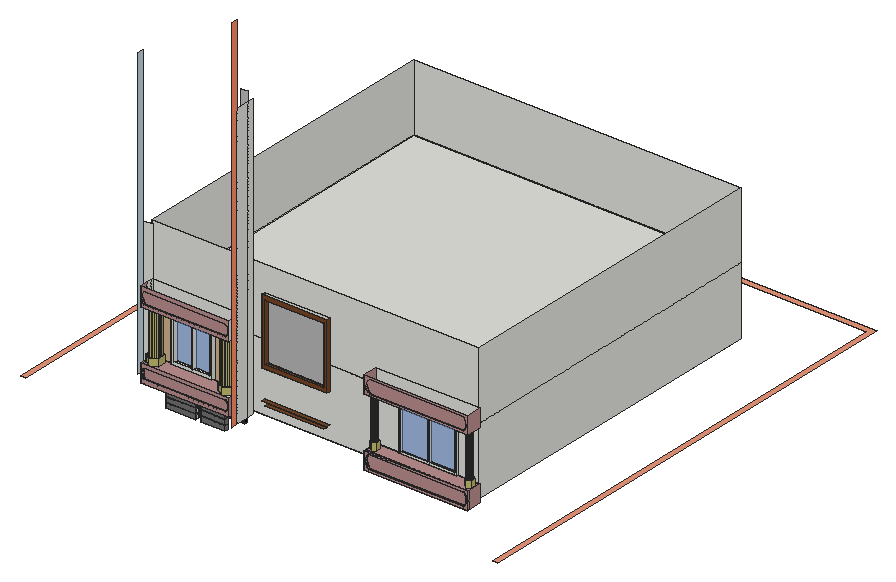
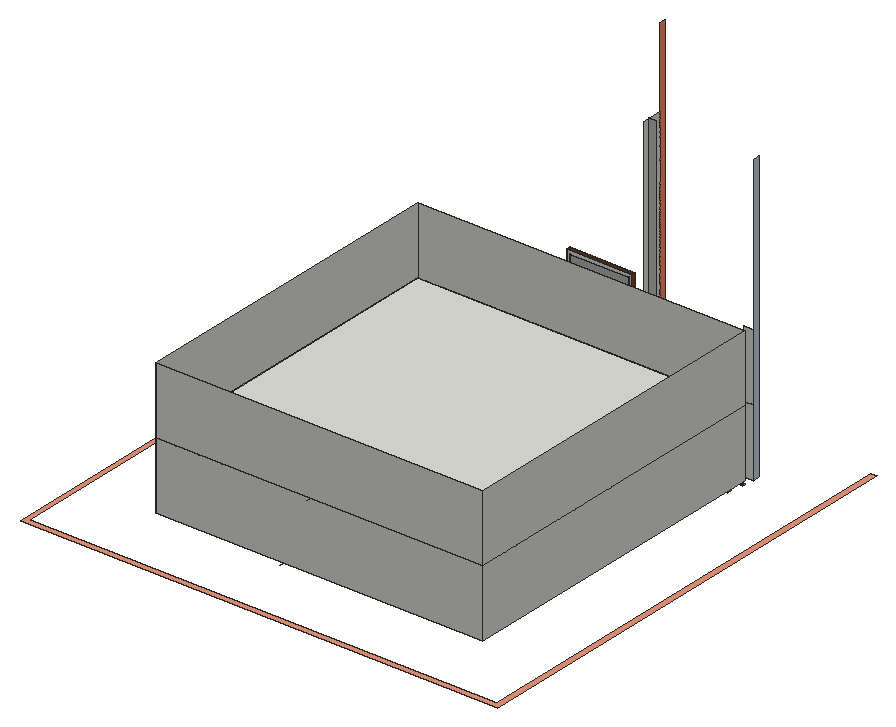
# SketchUp Ruby script. Lengths in inches.
U = 1.inch
M = Sketchup.active_model
def pt(a) = Geom::Point3d.new(a.map { |v| v * U })
def face(e, loops, mat)
  f = e.add_face(loops[0].map { |a| pt(a) })
  loops[1..].each { |l| e.add_face(l.map { |a| pt(a) }).erase! }
  f.material = f.back_material = mat if mat
  f
end
# faces: each face lists its corners as indices into pts; further lists are holes
def faces(e, pts, list, mat = nil) = list.each { |f| face(e, (f[0].is_a?(Array) ? f : [f]).map { |l| l.map { |i| pts[i] } }, mat) }
# xy, xz, yz: faces in a plane at the given z, y or x. An outline is a flat list of corners, or four numbers for a rectangle; further outlines are holes
def ring(l) = l.size == 4 ? [[l[0], l[1]], [l[2], l[1]], [l[2], l[3]], [l[0], l[3]]] : l.each_slice(2).to_a
def flat(e, list, mat, &to3) = list.each { |f| face(e, (f[0].is_a?(Array) ? f : [f]).map { |l| ring(l).map { |u, v| to3.(u, v) } }, mat) }
def xy(e, z, list, mat = nil) = flat(e, list, mat) { |x, y| [x, y, z] }
def xz(e, y, list, mat = nil) = flat(e, list, mat) { |x, z| [x, y, z] }
def yz(e, x, list, mat = nil) = flat(e, list, mat) { |y, z| [x, y, z] }
def lines(e, pts, list) = list.each { |a, b| e.add_line(pt(pts[a]), pt(pts[b])) }
# prism: a flat outline (further loops are holes) pulled along v
def prism(e, loops, v, mat = nil)
  f = face(e, loops, mat); d = Geom::Vector3d.new(v.map { |x| x * U })
  f.pushpull(f.normal.samedirection?(d) ? d.length : -d.length)
end
def box(e, o, s, mat = nil) = prism(e, [[o, [o[0] + s[0], o[1], o[2]], [o[0] + s[0], o[1] + s[1], o[2]], [o[0], o[1] + s[1], o[2]]]], [0, 0, s[2]], mat)
def at(x, y, z, deg = 0) = Geom::Transformation.translation(pt([x, y, z])) * Geom::Transformation.rotation(ORIGIN, Z_AXIS, deg.degrees)
def axes(o, x, y, z) = Geom::Transformation.new([*x, 0, *y, 0, *z, 0, *pt(o).to_a, 1])
def part(name) = M.definitions.add(name)
# library, detail: a bought-in or finely detailed component or shape, given as its bounding box
def library(name, o, s) = part(name).tap { |d| box(d.entities, o, s) }
def detail(e, o, s) = box(e.add_group.entities, o, s)
def put(e, d, t, mat = nil) = e.add_instance(d, t).tap { |i| i.material = mat if mat }
def group(e, t, mat = nil) = e.add_group.tap { |g| g.transformation = t; g.material = mat if mat }.entities
root = M.entities
M.materials.add("[0014_DarkSalmon]").color = [233, 150, 122]
M.materials.add("[0035_Tan]").color = [210, 180, 140]
M.materials.add("[0057_DarkKhaki]").color = [189, 183, 107]
M.materials.add("[0119_RosyBrown]").color = [188, 143, 143]
M.materials.add("[0131_Silver]").color = [192, 192, 192]
M.materials.add("[Color B03]").color = [255, 140, 101]
M.materials.add("[Color M05]").color = [114, 114, 114]
M.materials.add("[Color M09]").color = [0, 0, 0]
M.materials.add("[Mirror 01]").color = [185, 185, 185]
M.materials.add("[Mirror 02]").color = [229, 229, 229]
M.materials.add("[Terrazzo Light Blue]").color = [196, 214, 227]
M.materials.add("[Translucent Glass Blue]").color = [100, 149, 237]
M.materials["[Translucent Glass Blue]"].alpha = 0.5
M.materials.add("[Wood Veneer 01]").color = [120, 70, 37]
xy(root,81.75,[[173.97,107.37,183.17,113.37],[183.17,107.37,226.48,113.37]])
xy(root,81.9375,[[235.11,107.37,278.99,113.37]])
xy(root,90.5625,[[173.97,107.37,226.48,113.37]])
xy(root,90.75,[[235.11,107.37,278.99,113.37]],"[Color M05]")
xy(root,91.5625,[[173.97,107.37,183.17,113.37],[183.17,107.37,226.48,113.37]])
xy(root,91.6875,[[235.11,107.37,278.99,113.37]])
xy(root,100.375,[[173.97,107.37,226.48,113.37]])
xy(root,100.5,[[235.11,107.37,278.99,113.37]],"[Color M05]")
xy(root,101.375,[[173.97,107.37,183.17,113.37],[183.17,107.37,226.48,113.37]])
xy(root,101.4375,[[235.11,107.37,278.99,113.37]])
xy(root,101.48,[[278.99,113.37,309.83,116.37]],"[Color M09]")
xy(root,103.06,[[278.99,113.37,309.83,116.37]],"[Color M09]")
xy(root,105.17,[[143.99,113.37,173.97,116.37]],"[Color M09]")
xy(root,106.75,[[143.99,113.37,173.97,116.37]],"[Color M09]")
xy(root,110.1875,[[173.97,107.37,226.48,113.37]])
xy(root,110.25,[[235.11,107.37,278.99,113.37]])
xy(root,111.1875,[[173.97,107.37,183.17,113.37],[183.17,107.37,226.48,113.37],[235.11,107.37,278.99,113.37]])
xy(root,111.39,[[588.01,113.37,626.32,116.37],[629.68,113.37,664.64,116.37]])
xy(root,114.39,[[585.01,113.37,667.64,116.37]])
xy(root,120,[[173.97,107.37,174.52,116.37],[174.52,107.37,226.48,107.37,226.48,110.37,235.11,110.37,235.11,113.37,278.99,113.37,278.99,116.37,174.52,116.37],[235.11,107.37,278.99,113.37],[142.36,113.37,143.68,116.37],[309.83,113.37,312.71,116.37],
  [134.37,125.37,716.37,707.37]])
xy(root,120,[[0,0,9,0,9,832.73,841.73,832.73,841.73,0,850.73,0,850.73,841.73,0,841.73]],"[0014_DarkSalmon]")
xy(root,120,[[143.68,89.37,173.97,116.37],[173.97,89.37,174.52,107.37],[174.52,89.37,174.52,107.37,226.48,107.37,226.48,110.37,235.11,110.37,235.11,107.37,278.99,107.37,278.99,89.37],[278.99,89.37,299.74,116.37],[540.59,89.37,725.37,92.37],
  [540.59,92.37,725.37,116.37]],"[0119_RosyBrown]")
xy(root,123,[[548.74,89.37,717.93,92.37]],"[0119_RosyBrown]")
xy(root,123.625,[[551.85,96.57,553.73,96.8125,555.48,97.54,556.98,98.69,558.13,100.19,558.85,101.94,559.1,103.82,558.85,105.69,558.13,107.44,556.98,108.94,555.48,110.1,553.73,110.82,551.85,111.07,549.98,110.82,548.23,110.1,546.72,108.94,545.57,107.44,544.85,105.69,544.6,103.82,544.85,101.94,545.57,100.19,546.72,98.69,548.23,97.54,549.98,96.8125]])
xy(root,125.69,[[173.97,89.37,174.52,92.37]])
xy(root,125.69,[[149.37,89.37,173.97,92.37],[174.52,89.37,278.99,92.37],[278.99,89.37,294.05,92.37]],"[0119_RosyBrown]")
xy(root,139.875,[[714.79,96.57,716.67,96.8125,718.41,97.54,719.92,98.69,721.07,100.19,721.79,101.94,722.04,103.82,721.79,105.69,721.07,107.44,719.92,108.94,718.41,110.1,716.67,110.82,714.79,111.07,712.91,110.82,711.16,110.1,709.66,108.94,708.51,107.44,707.79,105.69,707.54,103.82,707.79,101.94,708.51,100.19,709.66,98.69,711.16,97.54,712.91,96.8125]])
xy(root,145.06,[[149.37,89.37,294.05,92.37]],"[0119_RosyBrown]")
xy(root,147.75,[[548.74,89.37,717.93,92.37]],"[0119_RosyBrown]")
xy(root,150.75,[[286.98,89.37,274.44,96.61,274.44,111.09,283.58,116.37,290.38,116.37,299.52,111.09,299.52,96.61],[286.98,89.37,299.74,89.37,299.74,116.37,290.38,116.37,299.52,111.09,299.52,96.61],[156.85,90.72,145.49,97.29,145.49,110.41,155.8,116.37,157.9,116.37,168.22,110.41,168.22,97.29],[548.7,96.13,542.32,99.82,542.32,107.19,548.7,110.88,555.09,107.19,555.09,99.82],[717.2,96.13,710.82,99.82,710.82,107.19,717.2,110.88,723.59,107.19,723.59,99.82],
  [155.8,116.37,157.9,116.37,156.85,116.97],[283.58,116.37,290.38,116.37,286.98,118.33]])
xy(root,150.75,[[143.68,89.37,286.98,89.37,274.44,96.61,274.44,111.09,283.58,116.37,157.9,116.37,168.22,110.41,168.22,97.29,156.85,90.72,145.49,97.29,145.49,110.41,155.8,116.37,143.68,116.37],[540.59,89.37,725.37,92.37],[[540.59,92.37,725.37,116.37],[548.7,96.13,542.32,99.82,542.32,107.19,548.7,110.88,555.09,107.19,555.09,99.82],[717.2,96.13,710.82,99.82,710.82,107.19,717.2,110.88,723.59,107.19,723.59,99.82]]],"[0119_RosyBrown]")
xy(root,151.69,[[583.77,113.37,686.39,116.37]])
xy(root,152.85,[[180.13,110.37,253.49,116.37]])
xy(root,154.69,[[586.77,113.37,635.08,116.37],[638.2,113.37,683.39,116.37]])
xy(root,157.74,[[185.03,110.37,216.81,116.37],[216.81,110.37,218.68,116.37],[218.68,110.37,248.59,116.37]])
xy(root,162.75,[[[286.98,89.37,299.52,96.61,299.52,111.09,290.38,116.37,283.58,116.37,274.44,111.09,274.44,96.61],[285.48,93.89,282.94,94.22,280.58,95.2,278.54,96.76,276.98,98.79,276,101.16,275.67,103.7,276,106.24,276.98,108.6,278.54,110.64,280.57,112.2,282.93,113.18,285.47,113.52,288.01,113.18,290.38,112.2,292.41,110.65,293.97,108.61,294.95,106.25,295.29,103.71,294.96,101.17,293.98,98.8,292.42,96.77,290.39,95.21,288.02,94.23]],[[156.85,90.72,168.22,97.29,168.22,110.41,157.9,116.37,155.8,116.37,145.49,110.41,145.49,97.29],[158.42,94,155.87,94.08,153.44,94.8125,151.27,96.15,149.53,98.01,148.32,100.25,147.74,102.73,147.82,105.27,148.55,107.71,149.89,109.875,151.75,111.62,153.99,112.82,156.47,113.4,159.01,113.33,161.45,112.59,163.61,111.25,165.36,109.4,166.5625,107.15,167.14,104.68,167.07,102.13,166.33,99.7,164.99,97.53,163.14,95.79,160.89,94.58]]])
xy(root,162.75,[[[548.7,96.13,555.09,99.82,555.09,107.19,548.7,110.88,542.32,107.19,542.32,99.82],[548.97,97.9,547.77,97.99,546.63,98.39,545.63,99.0625,544.84,99.98,544.3125,101.0625,544.09,102.25,544.17,103.45,544.57,104.59,545.25,105.59,546.16,106.38,547.25,106.91,548.43,107.14,549.64,107.05,550.78,106.66,551.78,105.98,552.57,105.06,553.09,103.98,553.32,102.79,553.23,101.59,552.84,100.45,552.16,99.45,551.25,98.66,550.16,98.13]],[[717.2,96.13,723.59,99.82,723.59,107.19,717.2,110.88,710.82,107.19,710.82,99.82],[717.54,97.9,716.33,97.99,715.19,98.39,714.19,99.0625,713.4,99.98,712.875,101.0625,712.65,102.25,712.74,103.45,713.13,104.59,713.81,105.59,714.72,106.38,715.81,106.91,716.99,107.14,718.2,107.05,719.34,106.66,720.34,105.98,721.13,105.06,721.66,103.98,721.88,102.79,721.8,101.59,721.4,100.45,720.72,99.45,719.81,98.66,718.72,98.13]]],"[0057_DarkKhaki]")
xy(root,170.74,[[376.4,74.37,481.09,80.37]],"[Wood Veneer 01]")
xy(root,176.74,[[370.4,74.37,487.09,80.37]],"[Wood Veneer 01]")
xy(root,230.12,[[370.4,74.37,487.09,80.37]],"[Wood Veneer 01]")
xy(root,231.13,[[586.77,113.37,635.08,116.37],[638.2,113.37,683.39,116.37]])
xy(root,233.05,[[185.03,110.37,216.81,116.37],[216.81,110.37,218.68,116.37],[218.68,110.37,248.59,116.37]])
xy(root,234.13,[[583.77,113.37,686.39,116.37]])
xy(root,236.12,[[376.4,74.37,481.09,80.37]],"[Wood Veneer 01]")
xy(root,237.95,[[180.13,110.37,253.49,116.37]])
xy(root,239.0625,[[285.48,93.89,288.02,94.23,290.39,95.21,292.42,96.77,293.98,98.8,294.96,101.17,295.29,103.71,294.95,106.25,293.97,108.61,292.41,110.65,290.38,112.2,288.01,113.18,285.47,113.52,282.93,113.18,280.57,112.2,278.54,110.64,276.98,108.6,276,106.24,275.67,103.7,276,101.16,276.98,98.79,278.54,96.76,280.58,95.2,282.94,94.22]])
xy(root,240,[[142.36,89.37,299.74,116.37],[158.42,94,160.89,94.58,163.14,95.79,164.99,97.53,166.33,99.7,167.07,102.13,167.14,104.68,166.5625,107.15,165.36,109.4,163.61,111.25,161.45,112.59,159.01,113.33,156.47,113.4,153.99,112.82,151.75,111.62,149.89,109.875,148.55,107.71,147.82,105.27,147.74,102.73,148.32,100.25,149.53,98.01,151.27,96.15,153.44,94.8125,155.87,94.08],[134.37,125.37,716.37,707.37]])
xy(root,240.5,[[540.59,89.37,725.37,116.37]],"[0119_RosyBrown]")
xy(root,243.5,[[548.97,97.9,550.16,98.13,551.25,98.66,552.16,99.45,552.84,100.45,553.23,101.59,553.32,102.79,553.09,103.98,552.57,105.06,551.78,105.98,550.78,106.66,549.64,107.05,548.43,107.14,547.25,106.91,546.16,106.38,545.25,105.59,544.57,104.59,544.17,103.45,544.09,102.25,544.3125,101.0625,544.84,99.98,545.63,99.0625,546.63,98.39,547.77,97.99],[717.54,97.9,718.72,98.13,719.81,98.66,720.72,99.45,721.4,100.45,721.8,101.59,721.88,102.79,721.66,103.98,721.13,105.06,720.34,105.98,719.34,106.66,718.2,107.05,716.99,107.14,715.81,106.91,714.72,106.38,713.81,105.59,713.13,104.59,712.74,103.45,712.65,102.25,712.875,101.0625,713.4,99.98,714.19,99.0625,715.19,98.39,716.33,97.99]])
xy(root,243.5,[[550.92,89.37,715.74,92.37]],"[0119_RosyBrown]")
xy(root,245.95,[[148.32,89.37,293.79,92.37]],"[0119_RosyBrown]")
xz(root,74.37,[[[370.4,230.12,487.09,346.81],[376.4,236.12,481.09,340.81]]],"[Wood Veneer 01]")
xz(root,80.37,[[[370.4,230.12,487.09,346.81],[376.4,236.12,481.09,340.81]]])
xz(root,80.37,[[376.4,236.12,481.09,340.81]],"[Mirror 01]")
xz(root,89.37,[[[143.68,120,299.74,150.75],[149.37,125.69,148.24,127.0625,147.3,128.57,146.55,130.17,146,131.86,145.67,133.6,145.56,135.375,145.67,137.15,146,138.89,146.55,140.58,147.3,142.18,148.24,143.6875,149.37,145.06,294.05,145.06,295.21,143.7,296.18,142.21,296.96,140.6,297.53,138.91,297.87,137.16,297.98,135.375,297.87,133.59,297.53,131.84,296.96,130.15,296.18,128.54,295.21,127.05,294.05,125.69]],[[540.59,120,725.37,150.75],[548.74,123,547.23,124.72,545.95,126.62,544.93,128.67,544.19,130.84,543.74,133.09,543.59,135.375,543.74,137.66,544.19,139.91,544.93,142.08,545.95,144.13,547.23,146.03,548.74,147.75,717.93,147.75,719.25,145.95,720.35,144,721.22,141.95,721.86,139.81,722.24,137.61,722.37,135.375,722.24,133.14,721.86,130.94,721.22,128.8,720.35,126.75,719.25,124.8,717.93,123]],[[142.36,240,299.74,272.875],[148.32,245.95,147.17,247.47,146.21,249.11,145.44,250.85,144.89,252.67,144.55,254.54,144.44,256.4375,144.55,258.34,144.89,260.21,145.44,262.03,146.21,263.77,147.17,265.41,148.32,266.92,293.79,266.92,295.16,265.51,296.32,263.92,297.25,262.18,297.93,260.33,298.34,258.4,298.47,256.4375,298.34,254.47,297.93,252.55,297.25,250.7,296.32,248.96,295.16,247.37,293.79,245.95]],[[540.59,240.5,725.37,271.25],[550.92,243.5,548.83,244.9,547.03,246.65,545.5625,248.69,544.48,250.95,543.82,253.375,543.59,255.875,543.82,258.375,544.48,260.8,545.5625,263.06,547.03,265.1,548.83,266.85,550.92,268.25,715.74,268.25,717.65,266.74,719.28,264.9375,720.6,262.9,721.58,260.66,722.17,258.3,722.37,255.875,722.17,253.45,721.58,251.09,720.6,248.85,719.28,246.8125,717.65,245.01,715.74,243.5]]],"[0119_RosyBrown]")
xz(root,92.37,[[[540.59,120,725.37,150.75],[548.74,123,717.93,123,719.25,124.8,720.35,126.75,721.22,128.8,721.86,130.94,722.24,133.14,722.37,135.375,722.24,137.61,721.86,139.81,721.22,141.95,720.35,144,719.25,145.95,717.93,147.75,548.74,147.75,547.23,146.03,545.95,144.13,544.93,142.08,544.19,139.91,543.74,137.66,543.59,135.375,543.74,133.09,544.19,130.84,544.93,128.67,545.95,126.62,547.23,124.72]]])
xz(root,92.37,[[548.74,123,717.93,123,719.25,124.8,720.35,126.75,721.22,128.8,721.86,130.94,722.24,133.14,722.37,135.375,722.24,137.61,721.86,139.81,721.22,141.95,720.35,144,719.25,145.95,717.93,147.75,548.74,147.75,547.23,146.03,545.95,144.13,544.93,142.08,544.19,139.91,543.74,137.66,543.59,135.375,543.74,133.09,544.19,130.84,544.93,128.67,545.95,126.62,547.23,124.72],[149.37,125.69,294.05,125.69,295.21,127.05,296.18,128.54,296.96,130.15,297.53,131.84,297.87,133.59,297.98,135.375,297.87,137.16,297.53,138.91,296.96,140.6,296.18,142.21,295.21,143.7,294.05,145.06,149.37,145.06,148.24,143.6875,147.3,142.18,146.55,140.58,146,138.89,145.67,137.15,145.56,135.375,145.67,133.6,146,131.86,146.55,130.17,147.3,128.57,148.24,127.0625],[550.92,243.5,715.74,243.5,717.65,245.01,719.28,246.8125,720.6,248.85,721.58,251.09,722.17,253.45,722.37,255.875,722.17,258.3,721.58,260.66,720.6,262.9,719.28,264.9375,717.65,266.74,715.74,268.25,550.92,268.25,548.83,266.85,547.03,265.1,545.5625,263.06,544.48,260.8,543.82,258.375,543.59,255.875,543.82,253.375,544.48,250.95,545.5625,248.69,547.03,246.65,548.83,244.9],[148.32,245.95,293.79,245.95,295.16,247.37,296.32,248.96,297.25,250.7,297.93,252.55,298.34,254.47,298.47,256.4375,298.34,258.4,297.93,260.33,297.25,262.18,296.32,263.92,295.16,265.51,293.79,266.92,148.32,266.92,147.17,265.41,146.21,263.77,145.44,262.03,144.89,260.21,144.55,258.34,144.44,256.4375,144.55,254.54,144.89,252.67,145.44,250.85,146.21,249.11,147.17,247.47]],"[0119_RosyBrown]")
xz(root,107.37,[[173.97,81.75,226.48,90.5625],[235.11,81.9375,278.99,90.75],[173.97,91.5625,226.48,100.375],[235.11,91.6875,278.99,100.5],[173.97,101.375,226.48,110.1875],
  [235.11,101.4375,278.99,110.25],[173.97,111.1875,226.48,120],[235.11,111.1875,278.99,120]],"[Color M05]")
xz(root,110.37,[[[180.13,152.85,253.49,237.95],[185.03,157.74,248.59,233.05]],[216.81,157.74,218.68,233.05]])
xz(root,113.37,[[173.97,81.75,183.17,90.5625],[183.17,81.75,226.48,90.5625],[235.11,81.9375,278.99,90.75],[173.97,90.5625,226.48,91.5625],[235.11,90.75,278.99,91.6875],
  [173.97,91.5625,183.17,100.375],[183.17,91.5625,226.48,100.375],[235.11,91.6875,278.99,100.5],[173.97,100.375,226.48,101.375],[235.11,100.5,278.99,101.4375],
  [173.97,101.375,183.17,110.1875],[183.17,101.375,226.48,110.1875],[235.11,101.4375,278.99,110.25],[173.97,110.1875,226.48,111.1875],[235.11,110.25,278.99,111.1875],
  [226.48,111.1875,227.05,120],[235.11,111.1875,278.99,120],[[583.77,151.69,686.39,234.13],[586.77,154.69,635.08,231.13],[638.2,154.69,683.39,231.13]]])
xz(root,113.37,[[278.99,101.48,309.83,103.06],[143.99,105.17,173.97,106.75]],"[Color M09]")
xz(root,116.37,[[278.99,101.48,309.83,103.06],[143.99,105.17,173.97,106.75],[173.97,105.17,174.52,106.75],[174.52,105.17,174.83,106.75],[173.97,106.75,174.52,120],
  [125.37,120,142.36,240],[143.68,120,299.74,150.75],[540.59,120,725.37,150.75],[155.8,150.75,157.9,162.75],[283.58,150.75,290.38,162.75],
  [[583.77,151.69,686.39,234.13],[586.77,154.69,635.08,231.13],[638.2,154.69,683.39,231.13]],[[180.13,152.85,253.49,237.95],[185.03,157.74,248.59,233.05]],[216.81,157.74,218.68,233.05],[125.37,240,142.36,360],[142.36,240,299.74,272.875],
  [540.59,240.5,725.37,271.25]])
xz(root,116.37,[[[142.36,120,143.68,120,143.68,150.75,155.8,150.75,155.8,162.75,157.9,162.75,157.9,150.75,283.58,150.75,283.58,162.75,290.38,162.75,290.38,150.75,299.74,150.75,299.74,240,142.36,240],[180.13,152.85,253.49,237.95]]],"[0035_Tan]")
xz(root,116.37,[[299.74,120,312.71,632]],"[0131_Silver]")
xz(root,116.37,[[278.99,103.06,309.83,120]],"[Mirror 02]")
xz(root,116.37,[[586.77,154.69,635.08,231.13],[638.2,154.69,683.39,231.13],[185.03,157.74,216.81,233.05],[218.68,157.74,248.59,233.05]],"[Translucent Glass Blue]")
xz(root,125.37,[[134.37,120,716.37,240],[134.37,240,716.37,360]])
xz(root,707.37,[[134.37,120,716.37,240],[134.37,240,716.37,360]])
yz(root,125.37,[[104.37,120,116.37,632]],"[Terrazzo Light Blue]")
yz(root,134.37,[[125.37,120,707.37,240],[125.37,240,707.37,360]])
yz(root,142.36,[[113.37,120,116.37,240],[104.37,240,113.37,272.875],[113.37,240,116.37,272.875]])
yz(root,142.36,[[89.37,240,104.37,272.875]],"[0119_RosyBrown]")
yz(root,143.68,[[89.37,120,116.37,150.75]],"[0119_RosyBrown]")
yz(root,143.99,[[113.37,105.17,116.37,106.75]])
yz(root,145.49,[[97.29,150.75,110.41,162.75]],"[0057_DarkKhaki]")
yz(root,168.22,[[97.29,150.75,110.41,162.75]],"[0057_DarkKhaki]")
yz(root,173.97,[[113.37,105.17,116.37,106.75],[113.37,106.75,116.37,120]])
yz(root,173.97,[[107.37,81.75,113.37,90.5625],[107.37,91.5625,113.37,100.375],[107.37,101.375,113.37,110.1875],[107.37,111.1875,113.37,120]],"[Color M05]")
yz(root,180.13,[[110.37,152.85,116.37,237.95]])
yz(root,185.03,[[110.37,157.74,116.37,233.05]])
yz(root,216.81,[[110.37,157.74,116.37,233.05]])
yz(root,218.68,[[110.37,157.74,116.37,233.05]])
yz(root,226.48,[[110.37,81.75,113.37,90.5625],[110.37,90.5625,113.37,91.5625],[110.37,91.5625,113.37,100.375],[110.37,100.375,113.37,101.375],[110.37,101.375,113.37,110.1875],
  [110.37,110.1875,113.37,111.1875],[110.37,111.1875,113.37,120]])
yz(root,226.48,[[107.37,81.75,110.37,90.5625],[107.37,91.5625,110.37,100.375],[107.37,101.375,110.37,110.1875],[107.37,111.1875,110.37,120]],"[Color M05]")
yz(root,235.11,[[110.37,81.9375,113.37,90.75],[110.37,90.75,113.37,91.6875],[110.37,91.6875,113.37,100.5],[110.37,100.5,113.37,101.4375],[110.37,101.4375,113.37,110.25],
  [110.37,110.25,113.37,111.1875],[110.37,111.1875,113.37,120]])
yz(root,235.11,[[107.37,81.9375,110.37,90.75],[107.37,91.6875,110.37,100.5],[107.37,101.4375,110.37,110.25],[107.37,111.1875,110.37,120]],"[Color M05]")
yz(root,248.59,[[110.37,157.74,116.37,233.05]])
yz(root,253.49,[[110.37,152.85,116.37,237.95]])
yz(root,274.44,[[96.61,150.75,111.09,162.75]],"[0057_DarkKhaki]")
yz(root,278.99,[[113.37,101.48,116.37,103.06]])
yz(root,278.99,[[107.37,81.9375,113.37,90.75],[107.37,91.6875,113.37,100.5],[107.37,101.4375,113.37,110.25],[113.37,103.06,116.37,120],[107.37,111.1875,113.37,120]],"[Color M05]")
yz(root,299.52,[[96.61,150.75,111.09,162.75]],"[0057_DarkKhaki]")
yz(root,299.74,[[89.37,240,116.37,272.875]])
yz(root,299.74,[[89.37,120,116.37,150.75]],"[0119_RosyBrown]")
yz(root,309.83,[[113.37,101.48,116.37,103.06]])
yz(root,309.83,[[113.37,103.06,116.37,120]],"[Color M09]")
yz(root,321.71,[[80.37,120,104.37,623],[104.37,120,116.37,623]])
yz(root,321.71,[[68.37,120,80.37,764.5625]],"[Color B03]")
yz(root,370.4,[[74.37,230.12,80.37,346.81]],"[Wood Veneer 01]")
yz(root,376.4,[[74.37,236.12,80.37,340.81]],"[Wood Veneer 01]")
yz(root,481.09,[[74.37,236.12,80.37,340.81]],"[Wood Veneer 01]")
yz(root,487.09,[[74.37,230.12,80.37,346.81]],"[Wood Veneer 01]")
yz(root,540.59,[[89.37,120,92.37,150.75],[92.37,120,116.37,150.75],[89.37,240.5,116.37,271.25]],"[0119_RosyBrown]")
yz(root,542.32,[[99.82,150.75,107.19,162.75]])
yz(root,555.09,[[99.82,150.75,107.19,162.75]],"[0057_DarkKhaki]")
yz(root,583.77,[[113.37,151.69,116.37,234.13]])
yz(root,586.77,[[113.37,154.69,116.37,231.13]])
yz(root,635.08,[[113.37,154.69,116.37,231.13]])
yz(root,638.2,[[113.37,154.69,116.37,231.13]])
yz(root,683.39,[[113.37,154.69,116.37,231.13]])
yz(root,686.39,[[113.37,151.69,116.37,234.13]])
yz(root,710.82,[[99.82,150.75,107.19,162.75]],"[0057_DarkKhaki]")
yz(root,716.37,[[125.37,120,707.37,240],[125.37,240,707.37,360]])
yz(root,723.59,[[99.82,150.75,107.19,162.75]],"[0057_DarkKhaki]")
yz(root,725.37,[[89.37,120,92.37,150.75],[92.37,120,116.37,150.75],[89.37,240.5,116.37,271.25]],"[0119_RosyBrown]")
p = [[548.74,92.37,123],[547.23,92.37,124.72],[547.23,89.37,124.72],[548.74,89.37,123],[719.25,92.37,124.8],[717.93,92.37,123],
  [717.93,89.37,123],[719.25,89.37,124.8],[545.95,92.37,126.62],[545.95,89.37,126.62],[720.35,92.37,126.75],[720.35,89.37,126.75],
  [149.37,92.37,125.69],[148.24,92.37,127.0625],[148.24,89.37,127.0625],[149.37,89.37,125.69],[295.21,92.37,127.05],[294.05,92.37,125.69],
  [294.05,89.37,125.69],[295.21,89.37,127.05],[544.93,92.37,128.67],[544.93,89.37,128.67],[721.22,92.37,128.8],[721.22,89.37,128.8],
  [296.18,92.37,128.54],[296.18,89.37,128.54],[147.3,92.37,128.57],[147.3,89.37,128.57],[296.96,92.37,130.15],[296.96,89.37,130.15],
  [146.55,92.37,130.17],[146.55,89.37,130.17],[544.19,92.37,130.84],[544.19,89.37,130.84],[721.86,92.37,130.94],[721.86,89.37,130.94],
  [297.53,92.37,131.84],[297.53,89.37,131.84],[146,92.37,131.86],[146,89.37,131.86],[543.74,92.37,133.09],[543.74,89.37,133.09],
  [722.24,92.37,133.14],[722.24,89.37,133.14],[297.87,92.37,133.59],[297.87,89.37,133.59],[145.67,92.37,133.6],[145.67,89.37,133.6],
  [543.59,92.37,135.375],[543.59,89.37,135.375],[722.37,92.37,135.375],[722.37,89.37,135.375],[145.56,92.37,135.375],[145.56,89.37,135.375],
  [297.98,92.37,135.375],[297.98,89.37,135.375],[145.67,92.37,137.15],[145.67,89.37,137.15],[297.87,92.37,137.16],[297.87,89.37,137.16],
  [543.74,92.37,137.66],[543.74,89.37,137.66],[722.24,92.37,137.61],[722.24,89.37,137.61],[146,92.37,138.89],[146,89.37,138.89],
  [297.53,92.37,138.91],[297.53,89.37,138.91],[721.86,92.37,139.81],[721.86,89.37,139.81],[544.19,92.37,139.91],[544.19,89.37,139.91],
  [146.55,92.37,140.58],[146.55,89.37,140.58],[296.96,92.37,140.6],[296.96,89.37,140.6],[721.22,92.37,141.95],[721.22,89.37,141.95],
  [544.93,92.37,142.08],[544.93,89.37,142.08],[147.3,92.37,142.18],[147.3,89.37,142.18],[296.18,92.37,142.21],[296.18,89.37,142.21],
  [720.35,92.37,144],[720.35,89.37,144],[545.95,92.37,144.13],[545.95,89.37,144.13],[148.24,92.37,143.6875],[148.24,89.37,143.6875],
  [295.21,92.37,143.7],[295.21,89.37,143.7],[149.37,92.37,145.06],[149.37,89.37,145.06],[294.05,92.37,145.06],[294.05,89.37,145.06],
  [719.25,92.37,145.95],[719.25,89.37,145.95],[547.23,92.37,146.03],[547.23,89.37,146.03],[717.93,92.37,147.75],[717.93,89.37,147.75],
  [548.74,92.37,147.75],[548.74,89.37,147.75],[274.44,96.61,150.75],[286.98,89.37,150.75],[286.98,89.37,162.75],[274.44,96.61,162.75],
  [299.52,96.61,150.75],[299.52,96.61,162.75],[145.49,97.29,150.75],[156.85,90.72,150.75],[156.85,90.72,162.75],[145.49,97.29,162.75],
  [168.22,97.29,150.75],[168.22,97.29,162.75],[542.32,99.82,150.75],[548.7,96.13,150.75],[548.7,96.13,162.75],[542.32,99.82,162.75],
  [555.09,99.82,150.75],[555.09,99.82,162.75],[710.82,99.82,150.75],[717.2,96.13,150.75],[717.2,96.13,162.75],[710.82,99.82,162.75],
  [723.59,99.82,150.75],[723.59,99.82,162.75],[548.7,110.88,150.75],[542.32,107.19,150.75],[542.32,107.19,162.75],[548.7,110.88,162.75],
  [555.09,107.19,150.75],[555.09,107.19,162.75],[717.2,110.88,150.75],[710.82,107.19,150.75],[710.82,107.19,162.75],[717.2,110.88,162.75],
  [723.59,107.19,150.75],[723.59,107.19,162.75],[155.8,116.37,150.75],[145.49,110.41,150.75],[145.49,110.41,162.75],[155.8,116.37,162.75],
  [168.22,110.41,150.75],[157.9,116.37,150.75],[157.9,116.37,162.75],[168.22,110.41,162.75],[283.58,116.37,150.75],[274.44,111.09,150.75],
  [274.44,111.09,162.75],[283.58,116.37,162.75],[299.52,111.09,150.75],[290.38,116.37,150.75],[290.38,116.37,162.75],[299.52,111.09,162.75],
  [282.94,94.22,162.75],[285.48,93.89,162.75],[285.48,93.89,239.0625],[282.94,94.22,239.0625],[288.02,94.23,162.75],[288.02,94.23,239.0625],
  [155.87,94.08,162.75],[158.42,94,162.75],[158.42,94,240],[155.87,94.08,240],[160.89,94.58,162.75],[160.89,94.58,240],
  [153.44,94.8125,162.75],[153.44,94.8125,240],[280.58,95.2,162.75],[280.58,95.2,239.0625],[290.39,95.21,162.75],[290.39,95.21,239.0625],
  [163.14,95.79,162.75],[163.14,95.79,240],[151.27,96.15,162.75],[151.27,96.15,240],[278.54,96.76,162.75],[278.54,96.76,239.0625],
  [292.42,96.77,162.75],[292.42,96.77,239.0625],[164.99,97.53,162.75],[164.99,97.53,240],[149.53,98.01,162.75],[149.53,98.01,240],
  [276.98,98.79,162.75],[276.98,98.79,239.0625],[293.98,98.8,162.75],[293.98,98.8,239.0625],[166.33,99.7,162.75],[166.33,99.7,240],
  [547.77,97.99,162.75],[548.97,97.9,162.75],[548.97,97.9,243.5],[547.77,97.99,243.5],[550.16,98.13,162.75],[550.16,98.13,243.5],
  [716.33,97.99,162.75],[717.54,97.9,162.75],[717.54,97.9,243.5],[716.33,97.99,243.5],[718.72,98.13,162.75],[718.72,98.13,243.5],
  [148.32,100.25,162.75],[148.32,100.25,240],[546.63,98.39,162.75],[546.63,98.39,243.5],[715.19,98.39,162.75],[715.19,98.39,243.5],
  [551.25,98.66,162.75],[551.25,98.66,243.5],[719.81,98.66,162.75],[719.81,98.66,243.5],[545.63,99.0625,162.75],[545.63,99.0625,243.5],
  [714.19,99.0625,162.75],[714.19,99.0625,243.5],[552.16,99.45,162.75],[552.16,99.45,243.5],[720.72,99.45,162.75],[720.72,99.45,243.5],
  [276,101.16,162.75],[276,101.16,239.0625],[294.96,101.17,162.75],[294.96,101.17,239.0625],[544.84,99.98,162.75],[544.84,99.98,243.5],
  [713.4,99.98,162.75],[713.4,99.98,243.5],[552.84,100.45,162.75],[552.84,100.45,243.5],[721.4,100.45,162.75],[721.4,100.45,243.5],
  [167.07,102.13,162.75],[167.07,102.13,240],[544.3125,101.0625,162.75],[544.3125,101.0625,243.5],[712.875,101.0625,162.75],[712.875,101.0625,243.5],
  [147.74,102.73,162.75],[147.74,102.73,240],[553.23,101.59,162.75],[553.23,101.59,243.5],[721.8,101.59,162.75],[721.8,101.59,243.5],
  [544.09,102.25,162.75],[544.09,102.25,243.5],[712.65,102.25,162.75],[712.65,102.25,243.5],[275.67,103.7,162.75],[275.67,103.7,239.0625],
  [295.29,103.71,162.75],[295.29,103.71,239.0625],[553.32,102.79,162.75],[553.32,102.79,243.5],[721.88,102.79,162.75],[721.88,102.79,243.5],
  [167.14,104.68,162.75],[167.14,104.68,240],[544.17,103.45,162.75],[544.17,103.45,243.5],[712.74,103.45,162.75],[712.74,103.45,243.5],
  [147.82,105.27,162.75],[147.82,105.27,240],[553.09,103.98,162.75],[553.09,103.98,243.5],[721.66,103.98,162.75],[721.66,103.98,243.5],
  [544.57,104.59,162.75],[544.57,104.59,243.5],[713.13,104.59,162.75],[713.13,104.59,243.5],[276,106.24,162.75],[276,106.24,239.0625],
  [294.95,106.25,162.75],[294.95,106.25,239.0625],[552.57,105.06,162.75],[552.57,105.06,243.5],[721.13,105.06,162.75],[721.13,105.06,243.5],
  [545.25,105.59,162.75],[545.25,105.59,243.5],[713.81,105.59,162.75],[713.81,105.59,243.5],[166.5625,107.15,162.75],[166.5625,107.15,240],
  [551.78,105.98,162.75],[551.78,105.98,243.5],[720.34,105.98,162.75],[720.34,105.98,243.5],[148.55,107.71,162.75],[148.55,107.71,240],
  [546.16,106.38,162.75],[546.16,106.38,243.5],[714.72,106.38,162.75],[714.72,106.38,243.5],[550.78,106.66,162.75],[550.78,106.66,243.5],
  [719.34,106.66,162.75],[719.34,106.66,243.5],[276.98,108.6,162.75],[276.98,108.6,239.0625],[293.97,108.61,162.75],[293.97,108.61,239.0625],
  [547.25,106.91,162.75],[547.25,106.91,243.5],[715.81,106.91,162.75],[715.81,106.91,243.5],[549.64,107.05,162.75],[549.64,107.05,243.5],
  [718.2,107.05,162.75],[718.2,107.05,243.5],[548.43,107.14,162.75],[548.43,107.14,243.5],[716.99,107.14,162.75],[716.99,107.14,243.5],
  [165.36,109.4,162.75],[165.36,109.4,240],[149.89,109.875,162.75],[149.89,109.875,240],[278.54,110.64,162.75],[278.54,110.64,239.0625],
  [292.41,110.65,162.75],[292.41,110.65,239.0625],[163.61,111.25,162.75],[163.61,111.25,240],[151.75,111.62,162.75],[151.75,111.62,240],
  [280.57,112.2,162.75],[280.57,112.2,239.0625],[290.38,112.2,162.75],[290.38,112.2,239.0625],[161.45,112.59,162.75],[161.45,112.59,240],
  [153.99,112.82,162.75],[153.99,112.82,240],[282.93,113.18,162.75],[282.93,113.18,239.0625],[288.01,113.18,162.75],[288.01,113.18,239.0625],
  [159.01,113.33,162.75],[159.01,113.33,240],[156.47,113.4,162.75],[156.47,113.4,240],[285.47,113.52,162.75],[285.47,113.52,239.0625],
  [550.92,92.37,243.5],[548.83,92.37,244.9],[548.83,89.37,244.9],[550.92,89.37,243.5],[717.65,92.37,245.01],[715.74,92.37,243.5],
  [715.74,89.37,243.5],[717.65,89.37,245.01],[547.03,92.37,246.65],[547.03,89.37,246.65],[719.28,92.37,246.8125],[719.28,89.37,246.8125],
  [148.32,92.37,245.95],[147.17,92.37,247.47],[147.17,89.37,247.47],[148.32,89.37,245.95],[295.16,92.37,247.37],[293.79,92.37,245.95],
  [293.79,89.37,245.95],[295.16,89.37,247.37],[545.5625,92.37,248.69],[545.5625,89.37,248.69],[720.6,92.37,248.85],[720.6,89.37,248.85],
  [296.32,92.37,248.96],[296.32,89.37,248.96],[146.21,92.37,249.11],[146.21,89.37,249.11],[544.48,92.37,250.95],[544.48,89.37,250.95],
  [721.58,92.37,251.09],[721.58,89.37,251.09],[297.25,92.37,250.7],[297.25,89.37,250.7],[145.44,92.37,250.85],[145.44,89.37,250.85],
  [297.93,92.37,252.55],[297.93,89.37,252.55],[144.89,92.37,252.67],[144.89,89.37,252.67],[543.82,92.37,253.375],[543.82,89.37,253.375],
  [722.17,92.37,253.45],[722.17,89.37,253.45],[298.34,92.37,254.47],[298.34,89.37,254.47],[144.55,92.37,254.54],[144.55,89.37,254.54],
  [543.59,92.37,255.875],[543.59,89.37,255.875],[722.37,92.37,255.875],[722.37,89.37,255.875],[183.17,113.37,120],[183.17,113.37,111.1875],
  [226.48,113.37,110.1875],[227.05,113.37,110.1875],[227.05,113.37,101.375],[226.48,113.37,101.375],[226.48,113.37,100.375],[227.05,113.37,100.375],
  [227.05,113.37,91.5625],[226.48,113.37,91.5625],[226.48,113.37,90.5625],[227.05,113.37,90.5625],[227.05,113.37,81.75],[226.48,113.37,81.75],
  [489.3,716.37,120],[489.3,707.37,120],[441.46,707.37,240],[441.46,716.37,240]]
faces(root,p,[[0,1,2,3],[4,5,6,7],[1,8,9,2],[10,4,7,11],[12,13,14,15],[16,17,18,19],[8,20,21,9],[22,10,11,23],
  [24,16,19,25],[13,26,27,14],[28,24,25,29],[26,30,31,27],[20,32,33,21],[34,22,23,35],[36,28,29,37],[30,38,39,31],
  [32,40,41,33],[42,34,35,43],[44,36,37,45],[38,46,47,39],[40,48,49,41],[50,42,43,51],[46,52,53,47],[54,44,45,55],
  [52,56,57,53],[58,54,55,59],[48,60,61,49],[62,50,51,63],[56,64,65,57],[66,58,59,67],[68,62,63,69],[60,70,71,61],
  [64,72,73,65],[74,66,67,75],[76,68,69,77],[70,78,79,71],[72,80,81,73],[82,74,75,83],[84,76,77,85],[78,86,87,79],
  [80,88,89,81],[90,82,83,91],[88,92,93,89],[94,90,91,95],[96,84,85,97],[86,98,99,87],[100,96,97,101],[98,102,103,99],
  [348,349,350,351],[352,353,354,355],[349,356,357,350],[358,352,355,359],[360,361,362,363],[364,365,366,367],[356,368,369,357],[370,358,359,371],
  [372,364,367,373],[361,374,375,362],[368,376,377,369],[378,370,371,379],[380,372,373,381],[374,382,383,375],[384,380,381,385],[382,386,387,383],
  [376,388,389,377],[390,378,379,391],[392,384,385,393],[386,394,395,387],[388,396,397,389],[398,390,391,399]],"[0119_RosyBrown]")
faces(root,p,[[104,105,106,107],[105,108,109,106],[110,111,112,113],[111,114,115,112],[116,117,118,119],[117,120,121,118],[122,123,124,125],[123,126,127,124],
  [132,128,131,133],[138,134,137,139],[156,157,158,159],[157,160,161,158],[162,163,164,165],[163,166,167,164],[168,162,165,169],[170,156,159,171],
  [160,172,173,161],[166,174,175,167],[176,168,169,177],[178,170,171,179],[172,180,181,173],[174,182,183,175],[184,176,177,185],[186,178,179,187],
  [180,188,189,181],[182,190,191,183],[192,193,194,195],[193,196,197,194],[198,199,200,201],[199,202,203,200],[204,184,185,205],[206,192,195,207],
  [208,198,201,209],[196,210,211,197],[202,212,213,203],[214,206,207,215],[216,208,209,217],[210,218,219,211],[212,220,221,213],[222,186,187,223],
  [188,224,225,189],[226,214,215,227],[228,216,217,229],[218,230,231,219],[220,232,233,221],[190,234,235,191],[236,226,227,237],[238,228,229,239],
  [240,204,205,241],[230,242,243,231],[232,244,245,233],[246,236,237,247],[248,238,239,249],[250,222,223,251],[224,252,253,225],[242,254,255,243],
  [244,256,257,245],[234,258,259,235],[260,246,247,261],[262,248,249,263],[264,240,241,265],[254,266,267,255],[256,268,269,257],[270,260,261,271],
  [272,262,263,273],[274,250,251,275],[252,276,277,253],[266,278,279,267],[268,280,281,269],[282,270,271,283],[284,272,273,285],[258,286,287,259],
  [278,288,289,279],[280,290,291,281],[292,264,265,293],[294,282,283,295],[296,284,285,297],[288,298,299,289],[290,300,301,291],[302,274,275,303],
  [276,304,305,277],[306,294,295,307],[308,296,297,309],[298,310,311,299],[300,312,313,301],[314,306,307,315],[316,308,309,317],[310,314,315,311],
  [312,316,317,313],[286,318,319,287],[320,292,293,321],[322,302,303,323],[304,324,325,305],[318,326,327,319],[328,320,321,329],[330,322,323,331],
  [324,332,333,325],[326,334,335,327],[336,328,329,337],[338,330,331,339],[332,340,341,333],[334,342,343,335],[344,336,337,345],[346,338,339,347],
  [340,346,347,341],[342,344,345,343]],"[0057_DarkKhaki]")
faces(root,p,[[128,129,130,131],[134,135,136,137],[140,141,142,143],[144,145,146,147],[148,149,150,151],[152,153,154,155]])
lines(root,p,[[400,401],[402,403],[404,405],[404,403],[406,407],[408,409],[408,407],[410,411],[412,413],[412,411],[414,415],[416,417]])
